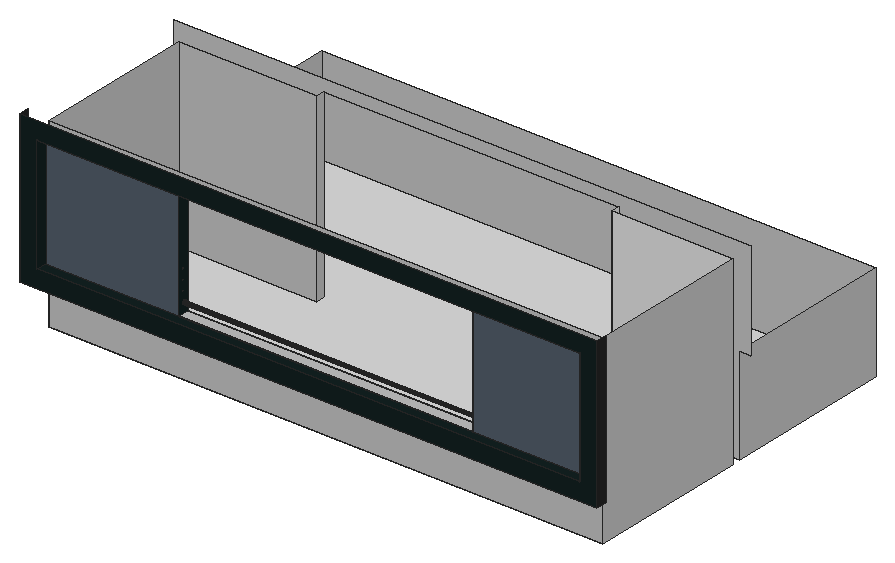
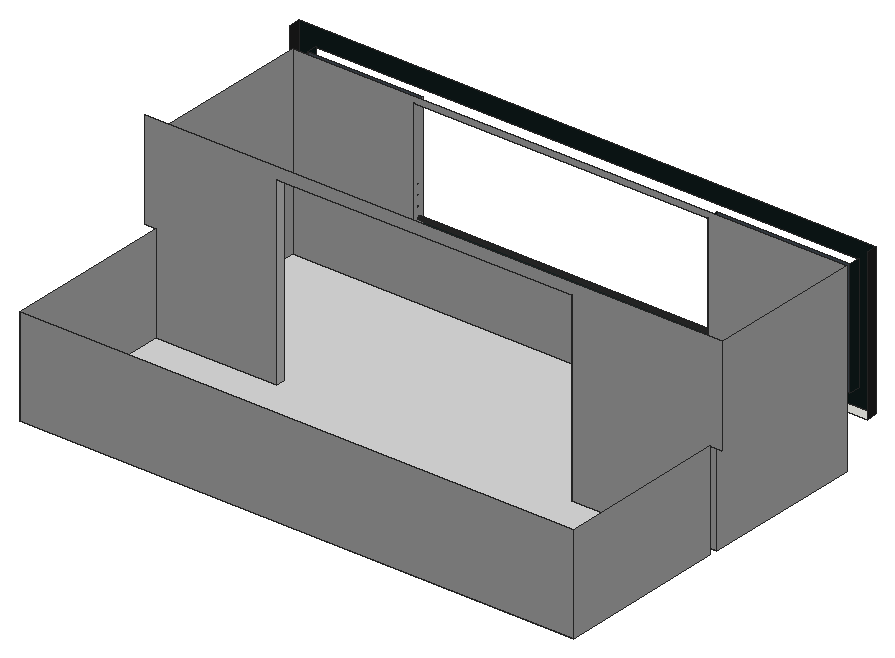
# SketchUp Ruby script. Lengths in millimetres.
U = 1.mm
M = Sketchup.active_model
def pt(a) = Geom::Point3d.new(a.map { |v| v * U })
def face(e, loops, mat)
  f = e.add_face(loops[0].map { |a| pt(a) })
  loops[1..].each { |l| e.add_face(l.map { |a| pt(a) }).erase! }
  f.material = f.back_material = mat if mat
  f
end
# faces: each face lists its corners as indices into pts; further lists are holes
def faces(e, pts, list, mat = nil) = list.each { |f| face(e, (f[0].is_a?(Array) ? f : [f]).map { |l| l.map { |i| pts[i] } }, mat) }
# xy, xz, yz: faces in a plane at the given z, y or x. An outline is a flat list of corners, or four numbers for a rectangle; further outlines are holes
def ring(l) = l.size == 4 ? [[l[0], l[1]], [l[2], l[1]], [l[2], l[3]], [l[0], l[3]]] : l.each_slice(2).to_a
def flat(e, list, mat, &to3) = list.each { |f| face(e, (f[0].is_a?(Array) ? f : [f]).map { |l| ring(l).map { |u, v| to3.(u, v) } }, mat) }
def xy(e, z, list, mat = nil) = flat(e, list, mat) { |x, y| [x, y, z] }
def xz(e, y, list, mat = nil) = flat(e, list, mat) { |x, z| [x, y, z] }
def yz(e, x, list, mat = nil) = flat(e, list, mat) { |y, z| [x, y, z] }
def lines(e, pts, list) = list.each { |a, b| e.add_line(pt(pts[a]), pt(pts[b])) }
# prism: a flat outline (further loops are holes) pulled along v
def prism(e, loops, v, mat = nil)
  f = face(e, loops, mat); d = Geom::Vector3d.new(v.map { |x| x * U })
  f.pushpull(f.normal.samedirection?(d) ? d.length : -d.length)
end
def box(e, o, s, mat = nil) = prism(e, [[o, [o[0] + s[0], o[1], o[2]], [o[0] + s[0], o[1] + s[1], o[2]], [o[0], o[1] + s[1], o[2]]]], [0, 0, s[2]], mat)
def at(x, y, z, deg = 0) = Geom::Transformation.translation(pt([x, y, z])) * Geom::Transformation.rotation(ORIGIN, Z_AXIS, deg.degrees)
def axes(o, x, y, z) = Geom::Transformation.new([*x, 0, *y, 0, *z, 0, *pt(o).to_a, 1])
def part(name) = M.definitions.add(name)
# library, detail: a bought-in or finely detailed component or shape, given as its bounding box
def library(name, o, s) = part(name).tap { |d| box(d.entities, o, s) }
def detail(e, o, s) = box(e.add_group.entities, o, s)
def put(e, d, t, mat = nil) = e.add_instance(d, t).tap { |i| i.material = mat if mat }
def group(e, t, mat = nil) = e.add_group.tap { |g| g.transformation = t; g.material = mat if mat }.entities
root = M.entities
M.materials.add("[0078_DarkSlateGray]").color = [19, 33, 33]
M.materials.add("[0111_SlateGray]").color = [81, 92, 104]
M.materials.add("[0130_Gainsboro]").color = [220, 220, 220]
M.materials.add("[0131_Silver]").color = [192, 192, 192]
M.materials.add("[0136_Charcoal]").color = [35, 35, 35]
xy(root,64811.3,[[7685.7,14719.3,36946.5,14719.3,36946.5,23253.7,30545.7,23253.7,30545.7,23710.9,36946.5,23710.9,36946.5,32702.5,7685.7,32702.5,7685.7,23710.9,15000.9,23710.9,15000.9,23253.7,7685.7,23253.7]],"[0130_Gainsboro]")
xy(root,67224.3,[[[7076.1,13550.9,37556.1,14109.7],[13199.6,13618.3,13223.5,13619.2,13247.2,13622.6,13270.4,13628.4,13292.9,13636.6,13314.4,13647.1,13334.6,13659.8,13353.5,13674.6,13370.7,13691.2,13386,13709.6,13399.4,13729.4,13410.6,13750.5,13419.5,13772.7,13426.1,13795.8,13430.2,13819.3,13431.8,13843.2,13431,13867.1,13427.6,13890.8,13421.8,13914,13413.6,13936.5,13403.1,13958,13390.4,13978.3,13375.6,13997.1,13359,14014.3,13340.6,14029.6,13320.8,14043,13299.6,14054.2,13277.4,14063.1,13254.4,14069.7,13230.9,14073.8,13207,14075.5,13183.1,14074.6,13159.4,14071.2,13136.2,14065.4,13113.7,14057.2,13092.2,14046.7,13071.9,14034,13053.1,14019.2,13035.9,14002.6,13020.5,13984.3,13007.2,13964.4,12996,13943.3,12987,13921.1,12980.5,13898,12976.3,13874.5,12974.7,13850.6,12975.6,13826.7,12978.9,13803,12984.7,13779.8,12993,13757.3,13003.5,13735.8,13016.2,13715.6,13030.9,13696.7,13047.6,13679.5,13065.9,13664.2,13085.8,13650.8,13106.9,13639.6,13129.1,13630.7,13152.1,13624.1,13175.7,13620],[21429.2,13618.3,21453.1,13619.2,21476.8,13622.6,21500,13628.4,21522.5,13636.6,21544,13647.1,21564.2,13659.8,21583.1,13674.6,21600.3,13691.2,21615.6,13709.6,21629,13729.4,21640.2,13750.5,21649.1,13772.7,21655.7,13795.8,21659.8,13819.3,21661.4,13843.2,21660.6,13867.1,21657.2,13890.8,21651.4,13914,21643.2,13936.5,21632.7,13958,21620,13978.3,21605.2,13997.1,21588.6,14014.3,21570.2,14029.6,21550.4,14043,21529.2,14054.2,21507,14063.1,21484,14069.7,21460.5,14073.8,21436.6,14075.5,21412.7,14074.6,21389,14071.2,21365.8,14065.4,21343.3,14057.2,21321.8,14046.7,21301.5,14034,21282.7,14019.2,21265.5,14002.6,21250.1,13984.3,21236.8,13964.4,21225.6,13943.3,21216.6,13921.1,21210.1,13898,21205.9,13874.5,21204.3,13850.6,21205.2,13826.7,21208.5,13803,21214.3,13779.8,21222.6,13757.3,21233.1,13735.8,21245.8,13715.6,21260.5,13696.7,21277.2,13679.5,21295.5,13664.2,21315.4,13650.8,21336.5,13639.6,21358.7,13630.7,21381.7,13624.1,21405.3,13620],[25086.8,13618.3,25110.7,13619.2,25134.4,13622.6,25157.6,13628.4,25180.1,13636.6,25201.6,13647.1,25221.8,13659.8,25240.7,13674.6,25257.9,13691.2,25273.2,13709.6,25286.6,13729.4,25297.8,13750.5,25306.7,13772.7,25313.3,13795.8,25317.4,13819.3,25319,13843.2,25318.2,13867.1,25314.8,13890.8,25309,13914,25300.8,13936.5,25290.3,13958,25277.6,13978.3,25262.8,13997.1,25246.2,14014.3,25227.8,14029.6,25208,14043,25186.8,14054.2,25164.6,14063.1,25141.6,14069.7,25118.1,14073.8,25094.2,14075.5,25070.3,14074.6,25046.6,14071.2,25023.4,14065.4,25000.9,14057.2,24979.4,14046.7,24959.1,14034,24940.3,14019.2,24923.1,14002.6,24907.7,13984.3,24894.4,13964.4,24883.2,13943.3,24874.2,13921.1,24867.7,13898,24863.5,13874.5,24861.9,13850.6,24862.8,13826.7,24866.1,13803,24871.9,13779.8,24880.2,13757.3,24890.7,13735.8,24903.4,13715.6,24918.1,13696.7,24934.8,13679.5,24953.1,13664.2,24973,13650.8,24994.1,13639.6,25016.3,13630.7,25039.3,13624.1,25062.9,13620],[32402,13618.3,32425.9,13619.2,32449.6,13622.6,32472.8,13628.4,32495.3,13636.6,32516.8,13647.1,32537,13659.8,32555.9,13674.6,32573.1,13691.2,32588.4,13709.6,32601.8,13729.4,32613,13750.5,32621.9,13772.7,32628.5,13795.8,32632.6,13819.3,32634.2,13843.2,32633.4,13867.1,32630,13890.8,32624.2,13914,32616,13936.5,32605.5,13958,32592.8,13978.3,32578,13997.1,32561.4,14014.3,32543,14029.6,32523.2,14043,32502,14054.2,32479.8,14063.1,32456.8,14069.7,32433.3,14073.8,32409.4,14075.5,32385.5,14074.6,32361.8,14071.2,32338.6,14065.4,32316.1,14057.2,32294.6,14046.7,32274.3,14034,32255.5,14019.2,32238.3,14002.6,32222.9,13984.3,32209.6,13964.4,32198.4,13943.3,32189.4,13921.1,32182.9,13898,32178.7,13874.5,32177.1,13850.6,32178,13826.7,32181.3,13803,32187.1,13779.8,32195.4,13757.3,32205.9,13735.8,32218.6,13715.6,32233.3,13696.7,32250,13679.5,32268.3,13664.2,32288.2,13650.8,32309.3,13639.6,32331.5,13630.7,32354.5,13624.1,32378.1,13620],[28744.4,13618.3,28768.3,13619.2,28792,13622.6,28815.2,13628.4,28837.7,13636.6,28859.2,13647.1,28879.4,13659.8,28898.3,13674.6,28915.5,13691.2,28930.8,13709.6,28944.2,13729.4,28955.4,13750.5,28964.3,13772.7,28970.9,13795.8,28975,13819.3,28976.6,13843.2,28975.8,13867.1,28972.4,13890.8,28966.6,13914,28958.4,13936.5,28947.9,13958,28935.2,13978.3,28920.4,13997.1,28903.8,14014.3,28885.4,14029.6,28865.6,14043,28844.4,14054.2,28822.2,14063.1,28799.2,14069.7,28775.7,14073.8,28751.8,14075.5,28727.9,14074.6,28704.2,14071.2,28681,14065.4,28658.5,14057.2,28637,14046.7,28616.7,14034,28597.9,14019.2,28580.7,14002.6,28565.3,13984.3,28552,13964.4,28540.8,13943.3,28531.8,13921.1,28525.3,13898,28521.1,13874.5,28519.5,13850.6,28520.4,13826.7,28523.7,13803,28529.5,13779.8,28537.8,13757.3,28548.3,13735.8,28561,13715.6,28575.7,13696.7,28592.4,13679.5,28610.7,13664.2,28630.6,13650.8,28651.7,13639.6,28673.9,13630.7,28696.9,13624.1,28720.5,13620],[36059.6,13618.3,36083.5,13619.2,36107.2,13622.6,36130.4,13628.4,36152.9,13636.6,36174.4,13647.1,36194.6,13659.8,36213.5,13674.6,36230.7,13691.2,36246,13709.6,36259.4,13729.4,36270.6,13750.5,36279.5,13772.7,36286.1,13795.8,36290.2,13819.3,36291.8,13843.2,36291,13867.1,36287.6,13890.8,36281.8,13914,36273.6,13936.5,36263.1,13958,36250.4,13978.3,36235.6,13997.1,36219,14014.3,36200.6,14029.6,36180.8,14043,36159.6,14054.2,36137.4,14063.1,36114.4,14069.7,36090.9,14073.8,36067,14075.5,36043.1,14074.6,36019.4,14071.2,35996.2,14065.4,35973.7,14057.2,35952.2,14046.7,35931.9,14034,35913.1,14019.2,35895.9,14002.6,35880.5,13984.3,35867.2,13964.4,35856,13943.3,35847,13921.1,35840.5,13898,35836.3,13874.5,35834.7,13850.6,35835.6,13826.7,35838.9,13803,35844.7,13779.8,35853,13757.3,35863.5,13735.8,35876.2,13715.6,35890.9,13696.7,35907.6,13679.5,35925.9,13664.2,35945.8,13650.8,35966.9,13639.6,35989.1,13630.7,36012.1,13624.1,36035.7,13620],[17771.6,13618.3,17795.5,13619.2,17819.2,13622.6,17842.4,13628.4,17864.9,13636.6,17886.4,13647.1,17906.6,13659.8,17925.5,13674.6,17942.7,13691.2,17958,13709.6,17971.4,13729.4,17982.6,13750.5,17991.5,13772.7,17998.1,13795.8,18002.2,13819.3,18003.8,13843.2,18003,13867.1,17999.6,13890.8,17993.8,13914,17985.6,13936.5,17975.1,13958,17962.4,13978.3,17947.6,13997.1,17931,14014.3,17912.6,14029.6,17892.8,14043,17871.6,14054.2,17849.4,14063.1,17826.4,14069.7,17802.9,14073.8,17779,14075.5,17755.1,14074.6,17731.4,14071.2,17708.2,14065.4,17685.7,14057.2,17664.2,14046.7,17643.9,14034,17625.1,14019.2,17607.9,14002.6,17592.5,13984.3,17579.2,13964.4,17568,13943.3,17559,13921.1,17552.5,13898,17548.3,13874.5,17546.7,13850.6,17547.6,13826.7,17550.9,13803,17556.7,13779.8,17565,13757.3,17575.5,13735.8,17588.2,13715.6,17602.9,13696.7,17619.6,13679.5,17637.9,13664.2,17657.8,13650.8,17678.9,13639.6,17701.1,13630.7,17724.1,13624.1,17747.7,13620]],[13199.6,13618.3,13175.7,13620,13152.1,13624.1,13129.1,13630.7,13106.9,13639.6,13085.8,13650.8,13065.9,13664.2,13047.6,13679.5,13030.9,13696.7,13016.2,13715.6,13003.5,13735.8,12993,13757.3,12984.7,13779.8,12978.9,13803,12975.6,13826.7,12974.7,13850.6,12976.3,13874.5,12980.5,13898,12987,13921.1,12996,13943.3,13007.2,13964.4,13020.5,13984.3,13035.9,14002.6,13053.1,14019.2,13071.9,14034,13092.2,14046.7,13113.7,14057.2,13136.2,14065.4,13159.4,14071.2,13183.1,14074.6,13207,14075.5,13230.9,14073.8,13254.4,14069.7,13277.4,14063.1,13299.6,14054.2,13320.8,14043,13340.6,14029.6,13359,14014.3,13375.6,13997.1,13390.4,13978.3,13403.1,13958,13413.6,13936.5,13421.8,13914,13427.6,13890.8,13431,13867.1,13431.8,13843.2,13430.2,13819.3,13426.1,13795.8,13419.5,13772.7,13410.6,13750.5,13399.4,13729.4,13386,13709.6,13370.7,13691.2,13353.5,13674.6,13334.6,13659.8,13314.4,13647.1,13292.9,13636.6,13270.4,13628.4,13247.2,13622.6,13223.5,13619.2],[17771.6,13618.3,17747.7,13620,17724.1,13624.1,17701.1,13630.7,17678.9,13639.6,17657.8,13650.8,17637.9,13664.2,17619.6,13679.5,17602.9,13696.7,17588.2,13715.6,17575.5,13735.8,17565,13757.3,17556.7,13779.8,17550.9,13803,17547.6,13826.7,17546.7,13850.6,17548.3,13874.5,17552.5,13898,17559,13921.1,17568,13943.3,17579.2,13964.4,17592.5,13984.3,17607.9,14002.6,17625.1,14019.2,17643.9,14034,17664.2,14046.7,17685.7,14057.2,17708.2,14065.4,17731.4,14071.2,17755.1,14074.6,17779,14075.5,17802.9,14073.8,17826.4,14069.7,17849.4,14063.1,17871.6,14054.2,17892.8,14043,17912.6,14029.6,17931,14014.3,17947.6,13997.1,17962.4,13978.3,17975.1,13958,17985.6,13936.5,17993.8,13914,17999.6,13890.8,18003,13867.1,18003.8,13843.2,18002.2,13819.3,17998.1,13795.8,17991.5,13772.7,17982.6,13750.5,17971.4,13729.4,17958,13709.6,17942.7,13691.2,17925.5,13674.6,17906.6,13659.8,17886.4,13647.1,17864.9,13636.6,17842.4,13628.4,17819.2,13622.6,17795.5,13619.2],[21429.2,13618.3,21405.3,13620,21381.7,13624.1,21358.7,13630.7,21336.5,13639.6,21315.4,13650.8,21295.5,13664.2,21277.2,13679.5,21260.5,13696.7,21245.8,13715.6,21233.1,13735.8,21222.6,13757.3,21214.3,13779.8,21208.5,13803,21205.2,13826.7,21204.3,13850.6,21205.9,13874.5,21210.1,13898,21216.6,13921.1,21225.6,13943.3,21236.8,13964.4,21250.1,13984.3,21265.5,14002.6,21282.7,14019.2,21301.5,14034,21321.8,14046.7,21343.3,14057.2,21365.8,14065.4,21389,14071.2,21412.7,14074.6,21436.6,14075.5,21460.5,14073.8,21484,14069.7,21507,14063.1,21529.2,14054.2,21550.4,14043,21570.2,14029.6,21588.6,14014.3,21605.2,13997.1,21620,13978.3,21632.7,13958,21643.2,13936.5,21651.4,13914,21657.2,13890.8,21660.6,13867.1,21661.4,13843.2,21659.8,13819.3,21655.7,13795.8,21649.1,13772.7,21640.2,13750.5,21629,13729.4,21615.6,13709.6,21600.3,13691.2,21583.1,13674.6,21564.2,13659.8,21544,13647.1,21522.5,13636.6,21500,13628.4,21476.8,13622.6,21453.1,13619.2],[25086.8,13618.3,25062.9,13620,25039.3,13624.1,25016.3,13630.7,24994.1,13639.6,24973,13650.8,24953.1,13664.2,24934.8,13679.5,24918.1,13696.7,24903.4,13715.6,24890.7,13735.8,24880.2,13757.3,24871.9,13779.8,24866.1,13803,24862.8,13826.7,24861.9,13850.6,24863.5,13874.5,24867.7,13898,24874.2,13921.1,24883.2,13943.3,24894.4,13964.4,24907.7,13984.3,24923.1,14002.6,24940.3,14019.2,24959.1,14034,24979.4,14046.7,25000.9,14057.2,25023.4,14065.4,25046.6,14071.2,25070.3,14074.6,25094.2,14075.5,25118.1,14073.8,25141.6,14069.7,25164.6,14063.1,25186.8,14054.2,25208,14043,25227.8,14029.6,25246.2,14014.3,25262.8,13997.1,25277.6,13978.3,25290.3,13958,25300.8,13936.5,25309,13914,25314.8,13890.8,25318.2,13867.1,25319,13843.2,25317.4,13819.3,25313.3,13795.8,25306.7,13772.7,25297.8,13750.5,25286.6,13729.4,25273.2,13709.6,25257.9,13691.2,25240.7,13674.6,25221.8,13659.8,25201.6,13647.1,25180.1,13636.6,25157.6,13628.4,25134.4,13622.6,25110.7,13619.2],
  [28744.4,13618.3,28720.5,13620,28696.9,13624.1,28673.9,13630.7,28651.7,13639.6,28630.6,13650.8,28610.7,13664.2,28592.4,13679.5,28575.7,13696.7,28561,13715.6,28548.3,13735.8,28537.8,13757.3,28529.5,13779.8,28523.7,13803,28520.4,13826.7,28519.5,13850.6,28521.1,13874.5,28525.3,13898,28531.8,13921.1,28540.8,13943.3,28552,13964.4,28565.3,13984.3,28580.7,14002.6,28597.9,14019.2,28616.7,14034,28637,14046.7,28658.5,14057.2,28681,14065.4,28704.2,14071.2,28727.9,14074.6,28751.8,14075.5,28775.7,14073.8,28799.2,14069.7,28822.2,14063.1,28844.4,14054.2,28865.6,14043,28885.4,14029.6,28903.8,14014.3,28920.4,13997.1,28935.2,13978.3,28947.9,13958,28958.4,13936.5,28966.6,13914,28972.4,13890.8,28975.8,13867.1,28976.6,13843.2,28975,13819.3,28970.9,13795.8,28964.3,13772.7,28955.4,13750.5,28944.2,13729.4,28930.8,13709.6,28915.5,13691.2,28898.3,13674.6,28879.4,13659.8,28859.2,13647.1,28837.7,13636.6,28815.2,13628.4,28792,13622.6,28768.3,13619.2],[32402,13618.3,32378.1,13620,32354.5,13624.1,32331.5,13630.7,32309.3,13639.6,32288.2,13650.8,32268.3,13664.2,32250,13679.5,32233.3,13696.7,32218.6,13715.6,32205.9,13735.8,32195.4,13757.3,32187.1,13779.8,32181.3,13803,32178,13826.7,32177.1,13850.6,32178.7,13874.5,32182.9,13898,32189.4,13921.1,32198.4,13943.3,32209.6,13964.4,32222.9,13984.3,32238.3,14002.6,32255.5,14019.2,32274.3,14034,32294.6,14046.7,32316.1,14057.2,32338.6,14065.4,32361.8,14071.2,32385.5,14074.6,32409.4,14075.5,32433.3,14073.8,32456.8,14069.7,32479.8,14063.1,32502,14054.2,32523.2,14043,32543,14029.6,32561.4,14014.3,32578,13997.1,32592.8,13978.3,32605.5,13958,32616,13936.5,32624.2,13914,32630,13890.8,32633.4,13867.1,32634.2,13843.2,32632.6,13819.3,32628.5,13795.8,32621.9,13772.7,32613,13750.5,32601.8,13729.4,32588.4,13709.6,32573.1,13691.2,32555.9,13674.6,32537,13659.8,32516.8,13647.1,32495.3,13636.6,32472.8,13628.4,32449.6,13622.6,32425.9,13619.2],[36059.6,13618.3,36035.7,13620,36012.1,13624.1,35989.1,13630.7,35966.9,13639.6,35945.8,13650.8,35925.9,13664.2,35907.6,13679.5,35890.9,13696.7,35876.2,13715.6,35863.5,13735.8,35853,13757.3,35844.7,13779.8,35838.9,13803,35835.6,13826.7,35834.7,13850.6,35836.3,13874.5,35840.5,13898,35847,13921.1,35856,13943.3,35867.2,13964.4,35880.5,13984.3,35895.9,14002.6,35913.1,14019.2,35931.9,14034,35952.2,14046.7,35973.7,14057.2,35996.2,14065.4,36019.4,14071.2,36043.1,14074.6,36067,14075.5,36090.9,14073.8,36114.4,14069.7,36137.4,14063.1,36159.6,14054.2,36180.8,14043,36200.6,14029.6,36219,14014.3,36235.6,13997.1,36250.4,13978.3,36263.1,13958,36273.6,13936.5,36281.8,13914,36287.6,13890.8,36291,13867.1,36291.8,13843.2,36290.2,13819.3,36286.1,13795.8,36279.5,13772.7,36270.6,13750.5,36259.4,13729.4,36246,13709.6,36230.7,13691.2,36213.5,13674.6,36194.6,13659.8,36174.4,13647.1,36152.9,13636.6,36130.4,13628.4,36107.2,13622.6,36083.5,13619.2]])
xy(root,68138.7,[[7990.5,13550.9,36641.7,14109.7]],"[0078_DarkSlateGray]")
xy(root,68138.7,[[15000.9,14109.7,30545.7,14719.3]],"[0131_Silver]")
xz(root,13550.9,[[[7076.1,67224.3,37556.1,75149.1],[7990.5,68138.7,36641.7,74234.7]]],"[0078_DarkSlateGray]")
xz(root,14109.7,[[15000.9,67224.3,30545.7,68138.7]])
xz(root,14109.7,[[7990.5,68138.7,15000.9,74234.7],[30545.7,68138.7,36641.7,74234.7]],"[0111_SlateGray]")
xz(root,14338.5,[[15000.9,68667.3,30545.7,68676.9]])
xz(root,14490.5,[[15000.9,68667.3,30545.7,68676.9]])
xz(root,14719.3,[[[7685.7,64811.3,36946.5,74539.5],[15000.9,68138.7,30545.7,74234.7]]],"[0131_Silver]")
xz(root,23253.7,[[30545.7,64811.3,36946.5,74539.5]],"[0130_Gainsboro]")
xz(root,23253.7,[[7685.7,64811.3,15000.9,74539.5]],"[0131_Silver]")
xz(root,23710.9,[[7685.7,64811.3,7685.7,69967.5,7076.1,69967.5,7076.1,75149.1,37556.1,75149.1,37556.1,69967.5,36946.5,69967.5,36946.5,64811.3,30545.7,64811.3,30545.7,74539.5,15000.9,74539.5,15000.9,64811.3]],"[0131_Silver]")
xz(root,32702.5,[[7685.7,64811.3,36946.5,69967.5]],"[0131_Silver]")
yz(root,7076.1,[[13550.9,67224.3,14109.7,75149.1]],"[0136_Charcoal]")
yz(root,7685.7,[[14719.3,64811.3,23253.7,74539.5],[23710.9,64811.3,32702.5,69967.5]],"[0131_Silver]")
yz(root,7990.5,[[13550.9,68138.7,14109.7,74234.7]],"[0078_DarkSlateGray]")
yz(root,15000.9,[[[14109.7,68138.7,14719.3,74234.7],[14414.5,70196.5,14404.9,70196.7,14395.5,70198.5,14386.4,70201.4,14377.8,70205.5,14369.7,70210.6,14362.3,70216.7,14355.8,70223.7,14350.2,70231.4,14345.6,70239.8,14342,70248.7,14339.6,70258,14338.5,70267.5,14338.5,70277.1,14339.6,70286.6,14342,70295.8,14345.6,70304.7,14350.2,70313.1,14355.8,70320.8,14362.3,70327.8,14369.7,70333.9,14377.8,70339,14386.4,70343.1,14395.5,70346.1,14404.9,70347.9,14414.5,70348.5,14424.1,70347.9,14433.5,70346.1,14442.6,70343.1,14451.2,70339,14459.3,70333.9,14466.7,70327.8,14473.2,70320.8,14478.8,70313.1,14483.4,70304.7,14487,70295.8,14489.4,70286.6,14490.5,70277.1,14490.5,70267.5,14489.4,70258,14487,70248.7,14483.4,70239.8,14478.8,70231.4,14473.2,70223.7,14466.7,70216.7,14459.3,70210.6,14451.2,70205.5,14442.6,70201.4,14433.5,70198.5,14424.1,70196.7],[14414.5,68596.3,14404.9,68596.5,14395.5,68598.3,14386.4,68601.2,14377.8,68605.3,14369.7,68610.4,14362.3,68616.5,14355.8,68623.5,14350.2,68631.2,14345.6,68639.6,14342,68648.5,14339.6,68657.8,14338.5,68667.3,14338.5,68676.9,14339.6,68686.4,14342,68695.6,14345.6,68704.5,14350.2,68712.9,14355.8,68720.6,14362.3,68727.6,14369.7,68733.7,14377.8,68738.8,14386.4,68742.9,14395.5,68745.9,14404.9,68747.7,14414.5,68748.3,14424.1,68747.7,14433.5,68745.9,14442.6,68742.9,14451.2,68738.8,14459.3,68733.7,14466.7,68727.6,14473.2,68720.6,14478.8,68712.9,14483.4,68704.5,14487,68695.6,14489.4,68686.4,14490.5,68676.9,14490.5,68667.3,14489.4,68657.8,14487,68648.5,14483.4,68639.6,14478.8,68631.2,14473.2,68623.5,14466.7,68616.5,14459.3,68610.4,14451.2,68605.3,14442.6,68601.2,14433.5,68598.3,14424.1,68596.5],[14414.5,69663.1,14404.9,69663.3,14395.5,69665.1,14386.4,69668,14377.8,69672.1,14369.7,69677.2,14362.3,69683.3,14355.8,69690.3,14350.2,69698,14345.6,69706.4,14342,69715.3,14339.6,69724.6,14338.5,69734.1,14338.5,69743.7,14339.6,69753.2,14342,69762.4,14345.6,69771.3,14350.2,69779.7,14355.8,69787.4,14362.3,69794.4,14369.7,69800.5,14377.8,69805.6,14386.4,69809.7,14395.5,69812.7,14404.9,69814.5,14414.5,69815.1,14424.1,69814.5,14433.5,69812.7,14442.6,69809.7,14451.2,69805.6,14459.3,69800.5,14466.7,69794.4,14473.2,69787.4,14478.8,69779.7,14483.4,69771.3,14487,69762.4,14489.4,69753.2,14490.5,69743.7,14490.5,69734.1,14489.4,69724.6,14487,69715.3,14483.4,69706.4,14478.8,69698,14473.2,69690.3,14466.7,69683.3,14459.3,69677.2,14451.2,69672.1,14442.6,69668,14433.5,69665.1,14424.1,69663.3],[14414.5,69129.7,14404.9,69129.9,14395.5,69131.7,14386.4,69134.6,14377.8,69138.7,14369.7,69143.8,14362.3,69149.9,14355.8,69156.9,14350.2,69164.6,14345.6,69173,14342,69181.9,14339.6,69191.2,14338.5,69200.7,14338.5,69210.3,14339.6,69219.8,14342,69229,14345.6,69237.9,14350.2,69246.3,14355.8,69254,14362.3,69261,14369.7,69267.1,14377.8,69272.2,14386.4,69276.3,14395.5,69279.3,14404.9,69281.1,14414.5,69281.7,14424.1,69281.1,14433.5,69279.3,14442.6,69276.3,14451.2,69272.2,14459.3,69267.1,14466.7,69261,14473.2,69254,14478.8,69246.3,14483.4,69237.9,14487,69229,14489.4,69219.8,14490.5,69210.3,14490.5,69200.7,14489.4,69191.2,14487,69181.9,14483.4,69173,14478.8,69164.6,14473.2,69156.9,14466.7,69149.9,14459.3,69143.8,14451.2,69138.7,14442.6,69134.6,14433.5,69131.7,14424.1,69129.9]]],"[0078_DarkSlateGray]")
yz(root,15000.9,[[23253.7,64811.3,23710.9,74539.5]],"[0131_Silver]")
yz(root,30545.7,[[23253.7,64811.3,23710.9,74539.5]],"[0130_Gainsboro]")
yz(root,30545.7,[[[14109.7,68138.7,14719.3,74234.7],[14414.5,70196.5,14424.1,70196.7,14433.5,70198.5,14442.6,70201.4,14451.2,70205.5,14459.3,70210.6,14466.7,70216.7,14473.2,70223.7,14478.8,70231.4,14483.4,70239.8,14487,70248.7,14489.4,70258,14490.5,70267.5,14490.5,70277.1,14489.4,70286.6,14487,70295.8,14483.4,70304.7,14478.8,70313.1,14473.2,70320.8,14466.7,70327.8,14459.3,70333.9,14451.2,70339,14442.6,70343.1,14433.5,70346.1,14424.1,70347.9,14414.5,70348.5,14404.9,70347.9,14395.5,70346.1,14386.4,70343.1,14377.8,70339,14369.7,70333.9,14362.3,70327.8,14355.8,70320.8,14350.2,70313.1,14345.6,70304.7,14342,70295.8,14339.6,70286.6,14338.5,70277.1,14338.5,70267.5,14339.6,70258,14342,70248.7,14345.6,70239.8,14350.2,70231.4,14355.8,70223.7,14362.3,70216.7,14369.7,70210.6,14377.8,70205.5,14386.4,70201.4,14395.5,70198.5,14404.9,70196.7],[14414.5,68596.3,14424.1,68596.5,14433.5,68598.3,14442.6,68601.2,14451.2,68605.3,14459.3,68610.4,14466.7,68616.5,14473.2,68623.5,14478.8,68631.2,14483.4,68639.6,14487,68648.5,14489.4,68657.8,14490.5,68667.3,14490.5,68676.9,14489.4,68686.4,14487,68695.6,14483.4,68704.5,14478.8,68712.9,14473.2,68720.6,14466.7,68727.6,14459.3,68733.7,14451.2,68738.8,14442.6,68742.9,14433.5,68745.9,14424.1,68747.7,14414.5,68748.3,14404.9,68747.7,14395.5,68745.9,14386.4,68742.9,14377.8,68738.8,14369.7,68733.7,14362.3,68727.6,14355.8,68720.6,14350.2,68712.9,14345.6,68704.5,14342,68695.6,14339.6,68686.4,14338.5,68676.9,14338.5,68667.3,14339.6,68657.8,14342,68648.5,14345.6,68639.6,14350.2,68631.2,14355.8,68623.5,14362.3,68616.5,14369.7,68610.4,14377.8,68605.3,14386.4,68601.2,14395.5,68598.3,14404.9,68596.5],[14414.5,69663.1,14424.1,69663.3,14433.5,69665.1,14442.6,69668,14451.2,69672.1,14459.3,69677.2,14466.7,69683.3,14473.2,69690.3,14478.8,69698,14483.4,69706.4,14487,69715.3,14489.4,69724.6,14490.5,69734.1,14490.5,69743.7,14489.4,69753.2,14487,69762.4,14483.4,69771.3,14478.8,69779.7,14473.2,69787.4,14466.7,69794.4,14459.3,69800.5,14451.2,69805.6,14442.6,69809.7,14433.5,69812.7,14424.1,69814.5,14414.5,69815.1,14404.9,69814.5,14395.5,69812.7,14386.4,69809.7,14377.8,69805.6,14369.7,69800.5,14362.3,69794.4,14355.8,69787.4,14350.2,69779.7,14345.6,69771.3,14342,69762.4,14339.6,69753.2,14338.5,69743.7,14338.5,69734.1,14339.6,69724.6,14342,69715.3,14345.6,69706.4,14350.2,69698,14355.8,69690.3,14362.3,69683.3,14369.7,69677.2,14377.8,69672.1,14386.4,69668,14395.5,69665.1,14404.9,69663.3],[14414.5,69129.7,14424.1,69129.9,14433.5,69131.7,14442.6,69134.6,14451.2,69138.7,14459.3,69143.8,14466.7,69149.9,14473.2,69156.9,14478.8,69164.6,14483.4,69173,14487,69181.9,14489.4,69191.2,14490.5,69200.7,14490.5,69210.3,14489.4,69219.8,14487,69229,14483.4,69237.9,14478.8,69246.3,14473.2,69254,14466.7,69261,14459.3,69267.1,14451.2,69272.2,14442.6,69276.3,14433.5,69279.3,14424.1,69281.1,14414.5,69281.7,14404.9,69281.1,14395.5,69279.3,14386.4,69276.3,14377.8,69272.2,14369.7,69267.1,14362.3,69261,14355.8,69254,14350.2,69246.3,14345.6,69237.9,14342,69229,14339.6,69219.8,14338.5,69210.3,14338.5,69200.7,14339.6,69191.2,14342,69181.9,14345.6,69173,14350.2,69164.6,14355.8,69156.9,14362.3,69149.9,14369.7,69143.8,14377.8,69138.7,14386.4,69134.6,14395.5,69131.7,14404.9,69129.9]]],"[0131_Silver]")
yz(root,36641.7,[[13550.9,68138.7,14109.7,74234.7]],"[0078_DarkSlateGray]")
yz(root,36946.5,[[14719.3,64811.3,23253.7,74539.5],[23710.9,64811.3,32702.5,69967.5]],"[0131_Silver]")
yz(root,37556.1,[[13550.9,67224.3,14109.7,75149.1]],"[0136_Charcoal]")
p = [[15000.9,14404.9,68596.5],[15000.9,14414.5,68596.3],[30545.7,14414.5,68596.3],[30545.7,14404.9,68596.5],[15000.9,14424.1,68596.5],[30545.7,14424.1,68596.5],
  [15000.9,14395.5,68598.3],[30545.7,14395.5,68598.3],[15000.9,14433.5,68598.3],[30545.7,14433.5,68598.3],[15000.9,14386.4,68601.2],[30545.7,14386.4,68601.2],
  [15000.9,14442.6,68601.2],[30545.7,14442.6,68601.2],[15000.9,14377.8,68605.3],[30545.7,14377.8,68605.3],[15000.9,14451.2,68605.3],[30545.7,14451.2,68605.3],
  [15000.9,14369.7,68610.4],[30545.7,14369.7,68610.4],[15000.9,14459.3,68610.4],[30545.7,14459.3,68610.4],[15000.9,14362.3,68616.5],[30545.7,14362.3,68616.5],
  [15000.9,14466.7,68616.5],[30545.7,14466.7,68616.5],[15000.9,14355.8,68623.5],[30545.7,14355.8,68623.5],[15000.9,14473.2,68623.5],[30545.7,14473.2,68623.5],
  [15000.9,14350.2,68631.2],[30545.7,14350.2,68631.2],[15000.9,14478.8,68631.2],[30545.7,14478.8,68631.2],[15000.9,14345.6,68639.6],[30545.7,14345.6,68639.6],
  [15000.9,14483.4,68639.6],[30545.7,14483.4,68639.6],[15000.9,14342,68648.5],[30545.7,14342,68648.5],[15000.9,14487,68648.5],[30545.7,14487,68648.5],
  [15000.9,14339.6,68657.8],[30545.7,14339.6,68657.8],[15000.9,14489.4,68657.8],[30545.7,14489.4,68657.8],[15000.9,14338.5,68667.3],[30545.7,14338.5,68667.3],
  [15000.9,14490.5,68667.3],[30545.7,14490.5,68667.3],[15000.9,14339.6,68686.4],[15000.9,14338.5,68676.9],[30545.7,14338.5,68676.9],[30545.7,14339.6,68686.4],
  [15000.9,14490.5,68676.9],[15000.9,14489.4,68686.4],[30545.7,14489.4,68686.4],[30545.7,14490.5,68676.9],[15000.9,14342,68695.6],[30545.7,14342,68695.6],
  [15000.9,14487,68695.6],[30545.7,14487,68695.6],[15000.9,14345.6,68704.5],[30545.7,14345.6,68704.5],[15000.9,14483.4,68704.5],[30545.7,14483.4,68704.5],
  [15000.9,14350.2,68712.9],[30545.7,14350.2,68712.9],[15000.9,14478.8,68712.9],[30545.7,14478.8,68712.9],[15000.9,14355.8,68720.6],[30545.7,14355.8,68720.6],
  [15000.9,14473.2,68720.6],[30545.7,14473.2,68720.6],[15000.9,14362.3,68727.6],[30545.7,14362.3,68727.6],[15000.9,14466.7,68727.6],[30545.7,14466.7,68727.6],
  [15000.9,14369.7,68733.7],[30545.7,14369.7,68733.7],[15000.9,14459.3,68733.7],[30545.7,14459.3,68733.7],[15000.9,14377.8,68738.8],[30545.7,14377.8,68738.8],
  [15000.9,14451.2,68738.8],[30545.7,14451.2,68738.8],[15000.9,14386.4,68742.9],[30545.7,14386.4,68742.9],[15000.9,14442.6,68742.9],[30545.7,14442.6,68742.9],
  [15000.9,14395.5,68745.9],[30545.7,14395.5,68745.9],[15000.9,14433.5,68745.9],[30545.7,14433.5,68745.9],[15000.9,14404.9,68747.7],[30545.7,14404.9,68747.7],
  [15000.9,14424.1,68747.7],[30545.7,14424.1,68747.7],[15000.9,14414.5,68748.3],[30545.7,14414.5,68748.3],[30545.7,14719.3,67224.3],[30545.7,14109.7,67224.3],
  [15000.9,14719.3,67224.3],[15000.9,14109.7,67224.3]]
faces(root,p,[[0,1,2,3],[1,4,5,2],[6,0,3,7],[4,8,9,5],[10,6,7,11],[8,12,13,9],[14,10,11,15],[12,16,17,13],
  [18,14,15,19],[16,20,21,17],[22,18,19,23],[20,24,25,21],[26,22,23,27],[24,28,29,25],[30,26,27,31],[28,32,33,29],
  [34,30,31,35],[32,36,37,33],[38,34,35,39],[36,40,41,37],[42,38,39,43],[40,44,45,41],[46,42,43,47],[44,48,49,45],
  [50,51,52,53],[54,55,56,57],[58,50,53,59],[55,60,61,56],[62,58,59,63],[60,64,65,61],[66,62,63,67],[64,68,69,65],
  [70,66,67,71],[68,72,73,69],[74,70,71,75],[72,76,77,73],[78,74,75,79],[76,80,81,77],[82,78,79,83],[80,84,85,81],
  [86,82,83,87],[84,88,89,85],[90,86,87,91],[88,92,93,89],[94,90,91,95],[92,96,97,93],[98,94,95,99],[96,98,99,97]])
lines(root,p,[[100,101],[102,103]])
